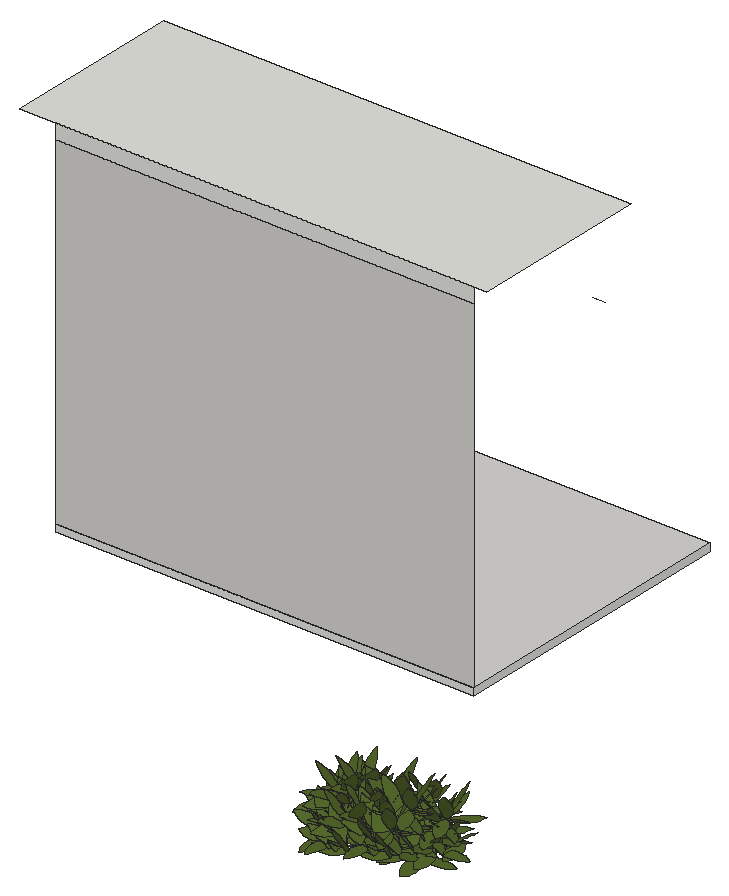
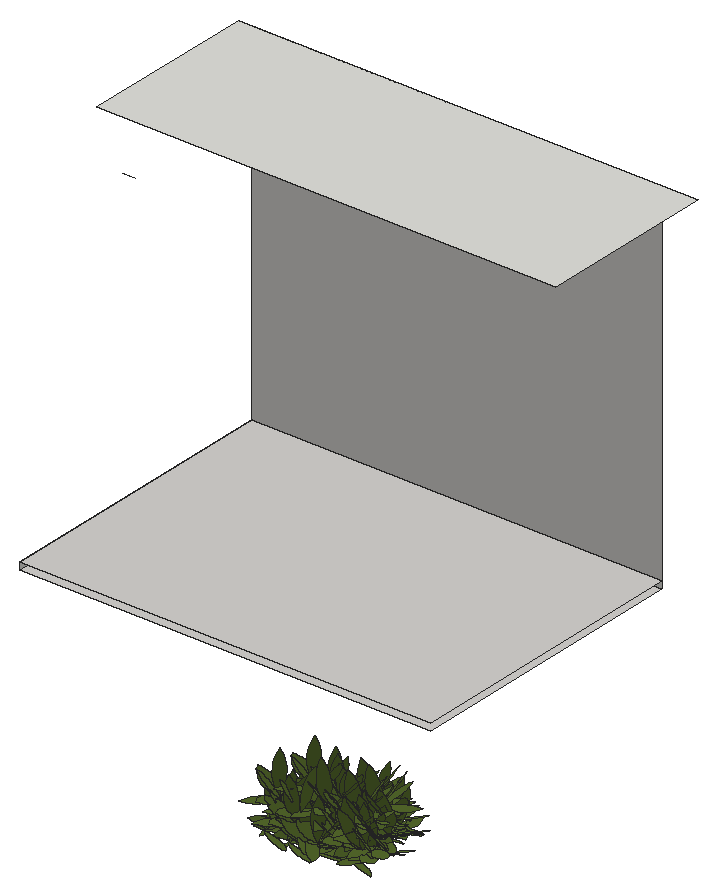
# SketchUp Ruby script. Lengths in inches.
U = 1.inch
M = Sketchup.active_model
def pt(a) = Geom::Point3d.new(a.map { |v| v * U })
def face(e, loops, mat)
  f = e.add_face(loops[0].map { |a| pt(a) })
  loops[1..].each { |l| e.add_face(l.map { |a| pt(a) }).erase! }
  f.material = f.back_material = mat if mat
  f
end
# faces: each face lists its corners as indices into pts; further lists are holes
def faces(e, pts, list, mat = nil) = list.each { |f| face(e, (f[0].is_a?(Array) ? f : [f]).map { |l| l.map { |i| pts[i] } }, mat) }
# xy, xz, yz: faces in a plane at the given z, y or x. An outline is a flat list of corners, or four numbers for a rectangle; further outlines are holes
def ring(l) = l.size == 4 ? [[l[0], l[1]], [l[2], l[1]], [l[2], l[3]], [l[0], l[3]]] : l.each_slice(2).to_a
def flat(e, list, mat, &to3) = list.each { |f| face(e, (f[0].is_a?(Array) ? f : [f]).map { |l| ring(l).map { |u, v| to3.(u, v) } }, mat) }
def xy(e, z, list, mat = nil) = flat(e, list, mat) { |x, y| [x, y, z] }
def xz(e, y, list, mat = nil) = flat(e, list, mat) { |x, z| [x, y, z] }
def yz(e, x, list, mat = nil) = flat(e, list, mat) { |y, z| [x, y, z] }
def lines(e, pts, list) = list.each { |a, b| e.add_line(pt(pts[a]), pt(pts[b])) }
# prism: a flat outline (further loops are holes) pulled along v
def prism(e, loops, v, mat = nil)
  f = face(e, loops, mat); d = Geom::Vector3d.new(v.map { |x| x * U })
  f.pushpull(f.normal.samedirection?(d) ? d.length : -d.length)
end
def box(e, o, s, mat = nil) = prism(e, [[o, [o[0] + s[0], o[1], o[2]], [o[0] + s[0], o[1] + s[1], o[2]], [o[0], o[1] + s[1], o[2]]]], [0, 0, s[2]], mat)
def at(x, y, z, deg = 0) = Geom::Transformation.translation(pt([x, y, z])) * Geom::Transformation.rotation(ORIGIN, Z_AXIS, deg.degrees)
def axes(o, x, y, z) = Geom::Transformation.new([*x, 0, *y, 0, *z, 0, *pt(o).to_a, 1])
def part(name) = M.definitions.add(name)
# library, detail: a bought-in or finely detailed component or shape, given as its bounding box
def library(name, o, s) = part(name).tap { |d| box(d.entities, o, s) }
def detail(e, o, s) = box(e.add_group.entities, o, s)
def put(e, d, t, mat = nil) = e.add_instance(d, t).tap { |i| i.material = mat if mat }
def group(e, t, mat = nil) = e.add_group.tap { |g| g.transformation = t; g.material = mat if mat }.entities
root = M.entities
M.materials.add("[0008_LavenderBlush]").color = [212, 210, 207]
M.materials.add("[Asphalt_New]").color = [85, 106, 44]
M.materials.add("white").color = [255, 255, 255]
c1 = part("Component\#59")
xy(c1.entities,0,[[5.79,0,4.75,0.06,3.73,0.22,2.73,0.5,1.77,0.88,0.86,1.37,0,1.95,0.83,2.59,1.74,3.13,2.7,3.56,3.7,3.87,4.74,4.05,5.79,4.12,6.84,4.05,7.87,3.87,8.88,3.56,9.84,3.13,10.74,2.59,11.57,1.95,10.72,1.37,9.8,0.88,8.84,0.5,7.84,0.22,6.82,0.06]],"[Asphalt_New]")
c2 = part("Leaf cluster")
put(c2.entities,c1,axes([10.37,9.23,1.73],[-0.67725,-0.67301,0.29729],[0.61625,-0.73963,-0.27052],[0.40195,0,0.91566]),"[Asphalt_New]")
put(c2.entities,c1,at(0,5.84,1.2),"[Asphalt_New]")
put(c2.entities,c1,axes([11.625,9.72,1.52],[-0.61694,-0.11161,0.77906],[-0.02647,-0.98639,-0.16227],[0.78657,-0.12073,0.60559]),"[Asphalt_New]")
put(c2.entities,c1,axes([13.35,8.05,1.98],[-0.1211,0.99122,-0.05316],[-0.90762,-0.13226,-0.39842],[-0.40195,0,0.91566]),"[Asphalt_New]")
c3 = part("Group141\#1")
p = [[0,0,0],[0,0,-2.45],[-0.68,0,-2.45],[4.45,-3.49,0],[-4.45,-3.49,0],[4.45,3.49,0],
  [4.45,0,0],[-4.45,3.49,0],[0.68,0,-2.45],[-4.45,0,0],[0,0,-3.97]]
lines(c3.entities,p,[[0,1],[1,2],[3,4],[5,6],[7,5],[1,8],[9,0],[0,6],[8,10],[4,9],[6,3],[2,10],
  [9,7]])
c4 = part("Rectangle Light")
put(c4.entities,c3,at(0,0,0))
xy(root,103.38,[[127.1875,9,148.875,24.3]],"[0008_LavenderBlush]")
xy(root,103.78,[[127.1875,9,148.875,24.3]],"[0008_LavenderBlush]")
xy(root,122.4375,[[125.3125,9,149.5625,18.35]])
xz(root,9,[[127.1875,103.38,148.875,103.78],[127.1875,121.625,148.875,122.4375]])
xz(root,9,[[127.1875,103.78,148.875,121.625]],"[0008_LavenderBlush]")
yz(root,148.875,[[9,103.38,24.3,103.78]])
p = [[148.875,16.67,118.57],[149.5625,16.67,118.57]]
lines(root,p,[[0,1]])
put(root,c1,axes([138.68,13.21,90.83],[0.01154,-0.09464,0.13861],[0.14952,-0.01265,-0.02887],[0.02521,0.11836,0.10775]),"[Asphalt_New]")
put(root,c1,axes([137.98,12,90.77],[0.00875,0.15182,0],[-0.15182,0.00875,0],[0,0,0.17792]),"[Asphalt_New]")
put(root,c1,axes([138.95,13.46,90.91],[-0.15155,-0.00971,-0.00946],[0.01213,-0.13895,-0.07089],[-0.00352,-0.06102,0.16292]),"[Asphalt_New]")
put(root,c1,axes([137.55,13.61,90.87],[0.09625,-0.10871,0.0529],[0.11768,0.08708,-0.04813],[0.00352,0.06102,0.16292]),"[Asphalt_New]")
put(root,c1,axes([137.45,12.3,90.56],[0.00875,0.15182,0],[-0.15182,0.00875,0],[0,0,0.17792]),"[Asphalt_New]")
put(root,c1,axes([137.49,13.8,90.83],[0.01154,-0.09464,0.13861],[0.14952,-0.01265,-0.02887],[0.02521,0.11836,0.10775]),"[Asphalt_New]")
put(root,c1,axes([139.68,12.39,90.99],[0.00875,0.15182,0],[-0.15182,0.00875,0],[0,0,0.17792]),"[Asphalt_New]")
put(root,c1,axes([140.28,13.99,90.83],[0.01154,-0.09464,0.13861],[0.14952,-0.01265,-0.02887],[0.02521,0.11836,0.10775]),"[Asphalt_New]")
put(root,c1,axes([137.02,13.91,90.65],[0.09625,-0.10871,0.0529],[0.11768,0.08708,-0.04813],[0.00352,0.06102,0.16292]),"[Asphalt_New]")
put(root,c1,axes([136.96,14.1,90.61],[0.01154,-0.09464,0.13861],[0.14952,-0.01265,-0.02887],[0.02521,0.11836,0.10775]),"[Asphalt_New]")
put(root,c2,axes([140.54,13.99,91.29],[-0.12016,0.09321,0],[-0.09321,-0.12016,0],[0,0,0.17792]),"white")
put(root,c1,axes([139.26,13.99,91.08],[0.09625,-0.10871,0.0529],[0.11768,0.08708,-0.04813],[0.00352,0.06102,0.16292]),"[Asphalt_New]")
put(root,c1,axes([139.19,14.19,91.04],[0.01154,-0.09464,0.13861],[0.14952,-0.01265,-0.02887],[0.02521,0.11836,0.10775]),"[Asphalt_New]")
put(root,c1,axes([139.41,12.8,90.77],[0.00875,0.15182,0],[-0.15182,0.00875,0],[0,0,0.17792]),"[Asphalt_New]")
put(root,c1,axes([137.76,14.05,90.91],[-0.15155,-0.00971,-0.00946],[0.01213,-0.13895,-0.07089],[-0.00352,-0.06102,0.16292]),"[Asphalt_New]")
put(root,c2,axes([137.56,12.1,91.42],[0.12994,0.079,0],[-0.079,0.12994,0],[0,0,0.17792]),"white")
put(root,c2,axes([141.87,13.48,91.41],[-0.06499,0.13748,0],[-0.13748,-0.06499,0],[0,0,0.17792]),"white")
put(root,c2,axes([136.61,13.25,90.73],[0.1271,-0.08349,0],[0.08349,0.1271,0],[0,0,0.17792]),"white")
put(root,c1,axes([139.68,14.6,91.41],[-0.12443,-0.07482,0.0529],[0.06418,-0.13158,-0.04813],[0.05936,-0.01458,0.16292]),"[Asphalt_New]")
put(root,c1,axes([140.55,14.24,90.91],[-0.15155,-0.00971,-0.00946],[0.01213,-0.13895,-0.07089],[-0.00352,-0.06102,0.16292]),"[Asphalt_New]")
put(root,c1,axes([138.98,14.4,90.87],[0.09625,-0.10871,0.0529],[0.11768,0.08708,-0.04813],[0.00352,0.06102,0.16292]),"[Asphalt_New]")
put(root,c1,axes([138.18,13.11,90.77],[0.00875,0.15182,0],[-0.15182,0.00875,0],[0,0,0.17792]),"[Asphalt_New]")
put(root,c1,axes([138.92,14.6,90.83],[0.01154,-0.09464,0.13861],[0.14952,-0.01265,-0.02887],[0.02521,0.11836,0.10775]),"[Asphalt_New]")
put(root,c1,axes([139.46,14.43,91.125],[-0.15155,-0.00971,-0.00946],[0.01213,-0.13895,-0.07089],[-0.00352,-0.06102,0.16292]),"[Asphalt_New]")
put(root,c1,axes([137.53,13.33,90.77],[0.00875,0.15182,0],[-0.15182,0.00875,0],[0,0,0.17792]),"[Asphalt_New]")
put(root,c1,axes([138.2,13.97,91.46],[0.15184,-0.00221,-0.00946],[-0.00119,0.13948,-0.07089],[0.0083,0.06056,0.16292]),"[Asphalt_New]")
put(root,c2,axes([141.41,13.92,91.41],[-0.06499,0.13748,0],[-0.13748,-0.06499,0],[0,0,0.17792]),"white")
put(root,c2,axes([138.25,15.96,90.87],[-0.12334,-0.08896,0],[0.08896,-0.12334,0],[0,0,0.17792]),"white")
put(root,c2,axes([140.5,14.72,90.51],[-0.12016,0.09321,0],[-0.09321,-0.12016,0],[0,0,0.17792]),"white")
put(root,c1,axes([137.76,14.71,90.87],[0.09625,-0.10871,0.0529],[0.11768,0.08708,-0.04813],[0.00352,0.06102,0.16292]),"[Asphalt_New]")
put(root,c1,axes([139.23,15.04,91.41],[-0.12443,-0.07482,0.0529],[0.06418,-0.13158,-0.04813],[0.05936,-0.01458,0.16292]),"[Asphalt_New]")
put(root,c1,axes([137.69,14.91,90.83],[0.01154,-0.09464,0.13861],[0.14952,-0.01265,-0.02887],[0.02521,0.11836,0.10775]),"[Asphalt_New]")
put(root,c1,axes([138.61,15.1875,91.18],[-0.09806,-0.10708,0.0529],[0.09891,-0.10794,-0.04813],[0.06106,0.00288,0.16292]),"[Asphalt_New]")
put(root,c1,axes([139.89,14.62,91.37],[-0.09516,0.0059,0.13861],[-0.03969,-0.14471,-0.02887],[0.11178,-0.04636,0.10775]),"[Asphalt_New]")
put(root,c2,axes([139.03,14.04,90.89],[-0.06499,0.13748,0],[-0.13748,-0.06499,0],[0,0,0.17792]),"white")
put(root,c2,axes([135.42,13.84,90.73],[0.1271,-0.08349,0],[0.08349,0.1271,0],[0,0,0.17792]),"white")
put(root,c2,axes([140.95,14.95,91.29],[-0.12303,0.08939,0],[-0.08939,-0.12303,0],[0,0,0.17792]),"white")
put(root,c2,axes([139.41,14.9,91.77],[-0.12016,0.09321,0],[-0.09321,-0.12016,0],[0,0,0.17792]),"white")
put(root,c1,axes([137.1,14.9375,90.87],[0.09625,-0.10871,0.0529],[0.11768,0.08708,-0.04813],[0.00352,0.06102,0.16292]),"[Asphalt_New]")
put(root,c1,axes([139.19,14.85,90.91],[-0.15155,-0.00971,-0.00946],[0.01213,-0.13895,-0.07089],[-0.00352,-0.06102,0.16292]),"[Asphalt_New]")
put(root,c2,axes([137.52,12.83,90.65],[0.12994,0.079,0],[-0.079,0.12994,0],[0,0,0.17792]),"white")
put(root,c2,axes([137.72,16.25,90.66],[-0.12334,-0.08896,0],[0.08896,-0.12334,0],[0,0,0.17792]),"white")
put(root,c1,axes([137.04,15.13,90.83],[0.01154,-0.09464,0.13861],[0.14952,-0.01265,-0.02887],[0.02521,0.11836,0.10775]),"[Asphalt_New]")
put(root,c1,axes([138.03,14.47,91.3125],[0.14768,-0.03627,0],[0.03627,0.14768,0],[0,0,0.17792]),"[Asphalt_New]")
put(root,c2,axes([141.01,14.73,91.18],[-0.10136,0.11337,0],[-0.11337,-0.10136,0],[0,0,0.17792]),"white")
put(root,c2,axes([138.21,14.03,90.73],[0.1271,-0.08349,0],[0.08349,0.1271,0],[0,0,0.17792]),"white")
put(root,c2,axes([142.32,14.29,92.12],[-0.06499,0.13748,0],[-0.13748,-0.06499,0],[0,0,0.17792]),"white")
put(root,c1,axes([138.04,15.48,91.18],[-0.09806,-0.10708,0.0529],[0.09891,-0.10794,-0.04813],[0.06106,0.00288,0.16292]),"[Asphalt_New]")
put(root,c2,axes([139.96,16.34,91.08],[-0.12334,-0.08896,0],[0.08896,-0.12334,0],[0,0,0.17792]),"white")
put(root,c2,axes([138.02,12.96,91.42],[0.12739,0.08305,0],[-0.08305,0.12739,0],[0,0,0.17792]),"white")
put(root,c2,axes([136.43,13.01,91.91],[0.12994,0.079,0],[-0.079,0.12994,0],[0,0,0.17792]),"white")
put(root,c1,axes([140.14,15.41,92.12],[-0.12443,-0.07482,0.0529],[0.06418,-0.13158,-0.04813],[0.05936,-0.01458,0.16292]),"[Asphalt_New]")
put(root,c1,axes([138.49,14.19,91.38],[-0.00408,0.09525,0.13861],[-0.14807,0.02435,-0.02887],[-0.03442,-0.11602,0.10775]),"[Asphalt_New]")
put(root,c1,axes([139.43,15.0625,91.37],[-0.09516,0.0059,0.13861],[-0.03969,-0.14471,-0.02887],[0.11178,-0.04636,0.10775]),"[Asphalt_New]")
put(root,c2,axes([137.13,14.22,90.95],[0.1271,-0.08349,0],[0.08349,0.1271,0],[0,0,0.17792]),"white")
put(root,c2,axes([138.56,15.26,91.0625],[-0.12016,0.09321,0],[-0.09321,-0.12016,0],[0,0,0.17792]),"white")
put(root,c1,axes([137.96,15.16,90.91],[-0.15155,-0.00971,-0.00946],[0.01213,-0.13895,-0.07089],[-0.00352,-0.06102,0.16292]),"[Asphalt_New]")
put(root,c1,axes([138.79,15.27,91.14],[-0.09292,-0.02137,0.13861],[0.00305,-0.15002,-0.02887],[0.12035,-0.0127,0.10775]),"[Asphalt_New]")
put(root,c1,axes([140.55,15.71,90.29],[0.01842,-0.15074,-0.00946],[0.13802,0.02011,-0.07089],[0.06112,0,0.16292]),"[Asphalt_New]")
put(root,c2,axes([140.45,15.03,91.18],[-0.10136,0.11337,0],[-0.11337,-0.10136,0],[0,0,0.17792]),"white")
put(root,c1,axes([139.51,15.73,90.5],[0.01842,-0.15074,-0.00946],[0.13802,0.02011,-0.07089],[0.06112,0,0.16292]),"[Asphalt_New]")
put(root,c1,axes([138.44,14.39,91.42],[-0.08742,0.11593,0.0529],[-0.12415,-0.07758,-0.04813],[-0.0083,-0.06056,0.16292]),"[Asphalt_New]")
put(root,c2,axes([140.89,13.39,90.11],[0.07604,0.1317,0],[-0.1317,0.07604,0],[0,0,0.17792]),"white")
put(root,c1,axes([137.05,14.6,91.08],[0.1519,0.00716,0],[-0.00716,0.1519,0],[0,0,0.17792]),"[Asphalt_New]")
put(root,c1,axes([138.16,14.6875,90.6875],[0.15184,-0.00221,-0.00946],[-0.00119,0.13948,-0.07089],[0.0083,0.06056,0.16292]),"[Asphalt_New]")
put(root,c2,axes([139.86,13.41,90.32],[0.07604,0.1317,0],[-0.1317,0.07604,0],[0,0,0.17792]),"white")
put(root,c2,axes([140.3,16.65,91.27],[-0.10525,-0.10976,0],[0.10976,-0.10525,0],[0,0,0.17792]),"white")
put(root,c1,axes([137.58,14.91,91.3125],[0.14768,-0.03627,0],[0.03627,0.14768,0],[0,0,0.17792]),"[Asphalt_New]")
put(root,c2,axes([139.6875,16.75,90.87],[-0.12334,-0.08896,0],[0.08896,-0.12334,0],[0,0,0.17792]),"white")
put(root,c1,axes([138.14,16.02,91.32],[-0.02064,-0.15066,0],[0.15066,-0.02064,0],[0,0,0.17792]),"[Asphalt_New]")
put(root,c1,axes([138.23,15.5625,91.14],[-0.09292,-0.02137,0.13861],[0.00305,-0.15002,-0.02887],[0.12035,-0.0127,0.10775]),"[Asphalt_New]")
put(root,c1,axes([138.61,14.85,91.46],[0.15183,0.00256,-0.00946],[-0.00557,0.13937,-0.07089],[0.00639,0.06079,0.16292]),"[Asphalt_New]")
put(root,c1,axes([137.07,14.875,91.95],[0.15184,-0.00221,-0.00946],[-0.00119,0.13948,-0.07089],[0.0083,0.06056,0.16292]),"[Asphalt_New]")
put(root,c2,axes([140.89,15.67,90.51],[-0.12303,0.08939,0],[-0.08939,-0.12303,0],[0,0,0.17792]),"white")
put(root,c1,axes([140.34,15.4375,92.08],[-0.09516,0.0059,0.13861],[-0.03969,-0.14471,-0.02887],[0.11178,-0.04636,0.10775]),"[Asphalt_New]")
put(root,c1,axes([140.08,14.3125,91.45],[0.01807,0.15078,-0.00946],[-0.13884,0.01339,-0.07089],[-0.05936,0.01458,0.16292]),"[Asphalt_New]")
put(root,c2,axes([136.85,14.64,90.73],[0.1271,-0.08349,0],[0.08349,0.1271,0],[0,0,0.17792]),"white")
put(root,c1,axes([136.49,14.89,91.08],[0.1519,0.00716,0],[-0.00716,0.1519,0],[0,0,0.17792]),"[Asphalt_New]")
put(root,c1,axes([138.81,16.09,91.89],[-0.09806,-0.10708,0.0529],[0.09891,-0.10794,-0.04813],[0.06106,0.00288,0.16292]),"[Asphalt_New]")
put(root,c2,axes([138.95,15.76,91.0625],[-0.12016,0.09321,0],[-0.09321,-0.12016,0],[0,0,0.17792]),"white")
put(root,c2,axes([139.79,15.82,91.77],[-0.12303,0.08939,0],[-0.08939,-0.12303,0],[0,0,0.17792]),"white")
put(root,c2,axes([138.46,17.0625,90.87],[-0.12334,-0.08896,0],[0.08896,-0.12334,0],[0,0,0.17792]),"white")
put(root,c1,axes([138.48,15.28,92.03],[0.14768,-0.03627,0],[0.03627,0.14768,0],[0,0,0.17792]),"[Asphalt_New]")
put(root,c2,axes([137.96,13.69,90.65],[0.12739,0.08305,0],[-0.08305,0.12739,0],[0,0,0.17792]),"white")
put(root,c2,axes([139.42,15.08,91.1],[-0.06499,0.13748,0],[-0.13748,-0.06499,0],[0,0,0.17792]),"white")
put(root,c2,axes([139.84,17.09,91.27],[-0.10525,-0.10976,0],[0.10976,-0.10525,0],[0,0,0.17792]),"white")
put(root,c1,axes([140.82,16.25,90.5],[0.01842,-0.15074,-0.00946],[0.13802,0.02011,-0.07089],[0.06112,0,0.16292]),"[Asphalt_New]")
put(root,c1,axes([140.45,14.56,91.3],[0.00875,0.15182,0],[-0.15182,0.00875,0],[0,0,0.17792]),"[Asphalt_New]")
put(root,c2,axes([141.22,15.64,91.89],[-0.10136,0.11337,0],[-0.11337,-0.10136,0],[0,0,0.17792]),"white")
put(root,c1,axes([137.24,16.19,91.1],[-0.12443,-0.07482,0.0529],[0.06418,-0.13158,-0.04813],[0.05936,-0.01458,0.16292]),"[Asphalt_New]")
put(root,c2,axes([141.16,13.93,90.32],[0.07604,0.1317,0],[-0.1317,0.07604,0],[0,0,0.17792]),"white")
put(root,c1,axes([136.21,15.24,91.24],[0.15184,-0.00221,-0.00946],[-0.00119,0.13948,-0.07089],[0.0083,0.06056,0.16292]),"[Asphalt_New]")
put(root,c1,axes([138.45,14.91,90.61],[-0.00408,0.09525,0.13861],[-0.14807,0.02435,-0.02887],[-0.03442,-0.11602,0.10775]),"[Asphalt_New]")
put(root,c2,axes([135.63,14.95,90.73],[0.1271,-0.08349,0],[0.08349,0.1271,0],[0,0,0.17792]),"white")
put(root,c2,axes([136.86,13.84,91.91],[0.12739,0.08305,0],[-0.08305,0.12739,0],[0,0,0.17792]),"white")
put(root,c2,axes([137.46,17.21,90.75],[-0.10525,-0.10976,0],[0.10976,-0.10525,0],[0,0,0.17792]),"white")
put(root,c1,axes([139.7,16.39,90.5],[0.01842,-0.15074,-0.00946],[0.13802,0.02011,-0.07089],[0.06112,0,0.16292]),"[Asphalt_New]")
put(root,c4,at(137.45,15.57,103.375,180))
put(root,c2,axes([137.81,17.29,90.87],[-0.12334,-0.08896,0],[0.08896,-0.12334,0],[0,0,0.17792]),"white")
put(root,c2,axes([139.875,15.27,90.89],[-0.06499,0.13748,0],[-0.13748,-0.06499,0],[0,0,0.17792]),"white")
put(root,c1,axes([138.4,15.11,90.64],[-0.08742,0.11593,0.0529],[-0.12415,-0.07758,-0.04813],[-0.0083,-0.06056,0.16292]),"[Asphalt_New]")
put(root,c2,axes([140.04,14.07,90.32],[0.07604,0.1317,0],[-0.1317,0.07604,0],[0,0,0.17792]),"white")
put(root,c2,axes([138.92,16.15,91.0625],[-0.12303,0.08939,0],[-0.08939,-0.12303,0],[0,0,0.17792]),"white")
put(root,c1,axes([139.625,14.76,91.45],[0.01807,0.15078,-0.00946],[-0.13884,0.01339,-0.07089],[-0.05936,0.01458,0.16292]),"[Asphalt_New]")
put(root,c2,axes([143.34,15.32,91.63],[-0.06499,0.13748,0],[-0.13748,-0.06499,0],[0,0,0.17792]),"white")
put(root,c1,axes([138.89,15.08,91.38],[-0.00707,0.09508,0.13861],[-0.14876,0.01968,-0.02887],[-0.03076,-0.11704,0.10775]),"[Asphalt_New]")
put(root,c1,axes([137.7,16.39,90.88],[-0.12443,-0.07482,0.0529],[0.06418,-0.13158,-0.04813],[0.05936,-0.01458,0.16292]),"[Asphalt_New]")
put(root,c2,axes([142.62,15.36,90.86],[-0.06499,0.13748,0],[-0.13748,-0.06499,0],[0,0,0.17792]),"white")
put(root,c1,axes([137.36,15.1,91.87],[-0.00408,0.09525,0.13861],[-0.14807,0.02435,-0.02887],[-0.03442,-0.11602,0.10775]),"[Asphalt_New]")
put(root,c1,axes([140.03,16.16,91.39],[0.09625,-0.10871,0.0529],[0.11768,0.08708,-0.04813],[0.00352,0.06102,0.16292]),"[Asphalt_New]")
put(root,c1,axes([142.58,16.04,90.15],[-0.15207,0,0],[0,-0.15207,0],[0,0,0.17792]),"[Asphalt_New]")
put(root,c2,axes([138.6,15.89,90.66],[-0.10136,0.11337,0],[-0.11337,-0.10136,0],[0,0,0.17792]),"white")
put(root,c1,axes([141.16,16.4375,91.63],[-0.12443,-0.07482,0.0529],[0.06418,-0.13158,-0.04813],[0.05936,-0.01458,0.16292]),"[Asphalt_New]")
put(root,c1,axes([138.99,16.18,91.85],[-0.09292,-0.02137,0.13861],[0.00305,-0.15002,-0.02887],[0.12035,-0.0127,0.10775]),"[Asphalt_New]")
put(root,c2,axes([134.98,15.17,90.73],[0.1271,-0.08349,0],[0.08349,0.1271,0],[0,0,0.17792]),"white")
put(root,c1,axes([141.54,16.07,90.36],[-0.15207,0,0],[0,-0.15207,0],[0,0,0.17792]),"[Asphalt_New]")
put(root,c1,axes([138.83,15.28,91.42],[-0.09102,0.11312,0.0529],[-0.12166,-0.08144,-0.04813],[-0.00639,-0.06079,0.16292]),"[Asphalt_New]")
put(root,c1,axes([140.43,16.48,90.86],[-0.12443,-0.07482,0.0529],[0.06418,-0.13158,-0.04813],[0.05936,-0.01458,0.16292]),"[Asphalt_New]")
put(root,c1,axes([137.25,14.88,90.93],[0.01807,0.15078,-0.00946],[-0.13884,0.01339,-0.07089],[-0.05936,0.01458,0.16292]),"[Asphalt_New]")
put(root,c1,axes([139.97,16.35,91.35],[0.01154,-0.09464,0.13861],[0.14952,-0.01265,-0.02887],[0.02521,0.11836,0.10775]),"[Asphalt_New]")
put(root,c2,axes([140.75,17.46,91.99],[-0.10525,-0.10976,0],[0.10976,-0.10525,0],[0,0,0.17792]),"white")
put(root,c2,axes([138.61,17.33,91.04],[-0.06975,-0.13513,0],[0.13513,-0.06975,0],[0,0,0.17792]),"white")
put(root,c1,axes([137.31,15.3,91.91],[-0.08742,0.11593,0.0529],[-0.12415,-0.07758,-0.04813],[-0.0083,-0.06056,0.16292]),"[Asphalt_New]")
put(root,c1,axes([138.1,16.75,90.55],[-0.02064,-0.15066,0],[0.15066,-0.02064,0],[0,0,0.17792]),"[Asphalt_New]")
put(root,c1,axes([139.07,15.03,91.22],[-0.0255,0.1497,-0.00946],[-0.13692,-0.02659,-0.07089],[-0.06106,-0.00288,0.16292]),"[Asphalt_New]")
put(root,c1,axes([137.26,15.5,91.79],[0.1519,0.00716,0],[-0.00716,0.1519,0],[0,0,0.17792]),"[Asphalt_New]")
put(root,c1,axes([140.8125,15.45,90.2],[0.09382,0.01697,0.13861],[0.00402,0.15,-0.02887],[-0.11961,0.01836,0.10775]),"[Asphalt_New]")
put(root,c1,axes([138.54,15.57,90.6875],[0.15183,0.00256,-0.00946],[-0.00557,0.13937,-0.07089],[0.00639,0.06079,0.16292]),"[Asphalt_New]")
put(root,c1,axes([139.78,15.48,90.42],[0.09382,0.01697,0.13861],[0.00402,0.15,-0.02887],[-0.11961,0.01836,0.10775]),"[Asphalt_New]")
put(root,c1,axes([136.59,16.76,91.25],[0.01842,-0.15074,-0.00946],[0.13802,0.02011,-0.07089],[0.06112,0,0.16292]),"[Asphalt_New]")
put(root,c1,axes([137.44,16.22,91.06],[-0.09516,0.0059,0.13861],[-0.03969,-0.14471,-0.02887],[0.11178,-0.04636,0.10775]),"[Asphalt_New]")
put(root,c1,axes([140.81,15.08,91.3],[0.00875,0.15182,0],[-0.15182,0.00875,0],[0,0,0.17792]),"[Asphalt_New]")
put(root,c1,axes([138.48,16.9,91.32],[-0.0159,-0.15124,0],[0.15124,-0.0159,0],[0,0,0.17792]),"[Asphalt_New]")
put(root,c1,axes([136.61,15.74,91.24],[0.15184,-0.00221,-0.00946],[-0.00119,0.13948,-0.07089],[0.0083,0.06056,0.16292]),"[Asphalt_New]")
put(root,c1,axes([137.01,16.93,91.8125],[-0.02064,-0.15066,0],[0.15066,-0.02064,0],[0,0,0.17792]),"[Asphalt_New]")
put(root,c1,axes([137.45,15.72,91.95],[0.15183,0.00256,-0.00946],[-0.00557,0.13937,-0.07089],[0.00639,0.06079,0.16292]),"[Asphalt_New]")
put(root,c1,axes([140.53,15.125,92.16],[0.01807,0.15078,-0.00946],[-0.13884,0.01339,-0.07089],[-0.05936,0.01458,0.16292]),"[Asphalt_New]")
put(root,c1,axes([137.3,16.9,90.47],[0.01842,-0.15074,-0.00946],[0.13802,0.02011,-0.07089],[0.06112,0,0.16292]),"[Asphalt_New]")
put(root,c2,axes([138.56,15.76,90.89],[-0.06499,0.13748,0],[-0.13748,-0.06499,0],[0,0,0.17792]),"white")
put(root,c2,axes([138.05,17.62,91.04],[-0.06975,-0.13513,0],[0.13513,-0.06975,0],[0,0,0.17792]),"white")
put(root,c1,axes([138.5,15.32,91.22],[-0.0255,0.1497,-0.00946],[-0.13692,-0.02659,-0.07089],[-0.06106,-0.00288,0.16292]),"[Asphalt_New]")
put(root,c2,axes([137.64,14.58,90.3],[0.07604,0.1317,0],[-0.1317,0.07604,0],[0,0,0.17792]),"white")
put(root,c1,axes([137.9,16.41,90.85],[-0.09516,0.0059,0.13861],[-0.03969,-0.14471,-0.02887],[0.11178,-0.04636,0.10775]),"[Asphalt_New]")
put(root,c2,axes([139.3,16.67,91.0625],[-0.12303,0.08939,0],[-0.08939,-0.12303,0],[0,0,0.17792]),"white")
put(root,c2,axes([138.62,16.09,90.24],[0.09591,-0.11801,0],[0.11801,0.09591,0],[0,0,0.17792]),"white")
put(root,c2,axes([137.58,16.11,90.46],[0.09591,-0.11801,0],[0.11801,0.09591,0],[0,0,0.17792]),"white")
put(root,c1,axes([141.36,16.46,91.59],[-0.09516,0.0059,0.13861],[-0.03969,-0.14471,-0.02887],[0.11178,-0.04636,0.10775]),"[Asphalt_New]")
put(root,c1,axes([140.64,16.5,90.82],[-0.09516,0.0059,0.13861],[-0.03969,-0.14471,-0.02887],[0.11178,-0.04636,0.10775]),"[Asphalt_New]")
put(root,c1,axes([140.38,16.6875,91.39],[0.09625,-0.10871,0.0529],[0.11768,0.08708,-0.04813],[0.00352,0.06102,0.16292]),"[Asphalt_New]")
put(root,c1,axes([140.24,16.6,91.44],[-0.15155,-0.00971,-0.00946],[0.01213,-0.13895,-0.07089],[-0.00352,-0.06102,0.16292]),"[Asphalt_New]")
put(root,c1,axes([139.93,15.38,92.01],[0.00875,0.15182,0],[-0.15182,0.00875,0],[0,0,0.17792]),"[Asphalt_New]")
put(root,c1,axes([142.84,16.59,90.36],[-0.15207,0,0],[0,-0.15207,0],[0,0,0.17792]),"[Asphalt_New]")
put(root,c2,axes([141.96,16.75,90.54],[-0.12016,0.09321,0],[-0.09321,-0.12016,0],[0,0,0.17792]),"white")
put(root,c1,axes([140.32,16.88,91.35],[0.01154,-0.09464,0.13861],[0.14952,-0.01265,-0.02887],[0.02521,0.11836,0.10775]),"[Asphalt_New]")
put(root,c1,axes([141,15.52,90.24],[0.10299,0.10235,0.0529],[-0.09371,0.11248,-0.04813],[-0.06112,0,0.16292]),"[Asphalt_New]")
put(root,c1,axes([136.04,16.26,90.79],[0.14768,-0.03627,0],[0.03627,0.14768,0],[0,0,0.17792]),"[Asphalt_New]")
put(root,c1,axes([136.58,16.05,91.24],[0.15183,0.00256,-0.00946],[-0.00557,0.13937,-0.07089],[0.00639,0.06079,0.16292]),"[Asphalt_New]")
put(root,c1,axes([138.79,17.2,90.625],[-0.09806,-0.10708,0.0529],[0.09891,-0.10794,-0.04813],[0.06106,0.00288,0.16292]),"[Asphalt_New]")
put(root,c1,axes([139.97,15.55,90.46],[0.10299,0.10235,0.0529],[-0.09371,0.11248,-0.04813],[-0.06112,0,0.16292]),"[Asphalt_New]")
put(root,c1,axes([138.82,15.48,90.75],[0.00875,0.15182,0],[-0.15182,0.00875,0],[0,0,0.17792]),"[Asphalt_New]")
put(root,c1,axes([138.82,15.8,90.61],[-0.00707,0.09508,0.13861],[-0.14876,0.01968,-0.02887],[-0.03076,-0.11704,0.10775]),"[Asphalt_New]")
put(root,c1,axes([141.08,16,90.42],[0.09382,0.01697,0.13861],[0.00402,0.15,-0.02887],[-0.11961,0.01836,0.10775]),"[Asphalt_New]")
put(root,c1,axes([139.5,16.3125,91.54],[0.14768,-0.03627,0],[0.03627,0.14768,0],[0,0,0.17792]),"[Asphalt_New]")
put(root,c1,axes([141.73,16.73,90.36],[-0.15207,0,0],[0,-0.15207,0],[0,0,0.17792]),"[Asphalt_New]")
put(root,c1,axes([138.78,16.35,90.76],[0.14768,-0.03627,0],[0.03627,0.14768,0],[0,0,0.17792]),"[Asphalt_New]")
put(root,c1,axes([138.77,16,90.64],[-0.09102,0.11312,0.0529],[-0.12166,-0.08144,-0.04813],[-0.00639,-0.06079,0.16292]),"[Asphalt_New]")
put(root,c1,axes([139.49,17.37,91.4],[-0.09806,-0.10708,0.0529],[0.09891,-0.10794,-0.04813],[0.06106,0.00288,0.16292]),"[Asphalt_New]")
put(root,c1,axes([139.5,16.98,92.1],[0.09625,-0.10871,0.0529],[0.11768,0.08708,-0.04813],[0.00352,0.06102,0.16292]),"[Asphalt_New]")
put(root,c1,axes([137.73,15.95,91.87],[-0.00707,0.09508,0.13861],[-0.14876,0.01968,-0.02887],[-0.03076,-0.11704,0.10775]),"[Asphalt_New]")
put(root,c1,axes([139.96,16.14,90.42],[0.09382,0.01697,0.13861],[0.00402,0.15,-0.02887],[-0.11961,0.01836,0.10775]),"[Asphalt_New]")
put(root,c2,axes([138.97,14.86,90.67],[0.12994,0.079,0],[-0.079,0.12994,0],[0,0,0.17792]),"white")
put(root,c1,axes([136.89,15.96,91.16],[-0.00408,0.09525,0.13861],[-0.14807,0.02435,-0.02887],[-0.03442,-0.11602,0.10775]),"[Asphalt_New]")
put(root,c2,axes([137.85,18.25,90.96],[-0.10525,-0.10976,0],[0.10976,-0.10525,0],[0,0,0.17792]),"white")
put(root,c2,axes([141.33,17.03,90.54],[-0.12016,0.09321,0],[-0.09321,-0.12016,0],[0,0,0.17792]),"white")
put(root,c2,axes([141.2,16.75,90.63],[-0.10136,0.11337,0],[-0.11337,-0.10136,0],[0,0,0.17792]),"white")
put(root,c1,axes([139.4375,17.18,92.06],[0.01154,-0.09464,0.13861],[0.14952,-0.01265,-0.02887],[0.02521,0.11836,0.10775]),"[Asphalt_New]")
put(root,c1,axes([138.4,17.08,90.84],[0.09625,-0.10871,0.0529],[0.11768,0.08708,-0.04813],[0.00352,0.06102,0.16292]),"[Asphalt_New]")
put(root,c1,axes([137.67,16.15,91.91],[-0.09102,0.11312,0.0529],[-0.12166,-0.08144,-0.04813],[-0.00639,-0.06079,0.16292]),"[Asphalt_New]")
put(root,c2,axes([135.8125,18.17,90.73],[-0.06975,-0.13513,0],[0.13513,-0.06975,0],[0,0,0.17792]),"white")
put(root,c1,axes([141.34,17.48,90.5],[0.01842,-0.15074,-0.00946],[0.13802,0.02011,-0.07089],[0.06112,0,0.16292]),"[Asphalt_New]")
put(root,c1,axes([138.34,17.28,90.8],[0.01154,-0.09464,0.13861],[0.14952,-0.01265,-0.02887],[0.02521,0.11836,0.10775]),"[Asphalt_New]")
put(root,c2,axes([138.8125,18.24,91.76],[-0.06975,-0.13513,0],[0.13513,-0.06975,0],[0,0,0.17792]),"white")
put(root,c2,axes([138.88,16.64,90.46],[0.09591,-0.11801,0],[0.11801,0.09591,0],[0,0,0.17792]),"white")
put(root,c1,axes([138.42,17.62,90.55],[-0.0159,-0.15124,0],[0.15124,-0.0159,0],[0,0,0.17792]),"[Asphalt_New]")
put(root,c2,axes([141.68,15.16,90.32],[0.07604,0.1317,0],[-0.1317,0.07604,0],[0,0,0.17792]),"white")
put(root,c1,axes([139.27,15.94,91.93],[-0.0255,0.1497,-0.00946],[-0.13692,-0.02659,-0.07089],[-0.06106,-0.00288,0.16292]),"[Asphalt_New]")
put(root,c2,axes([140.4,16.42,90.89],[-0.06499,0.13748,0],[-0.13748,-0.06499,0],[0,0,0.17792]),"white")
put(root,c2,axes([138.31,18.4375,90.75],[-0.10525,-0.10976,0],[0.10976,-0.10525,0],[0,0,0.17792]),"white")
put(root,c2,axes([141.9,16.92,91.4],[-0.10136,0.11337,0],[-0.11337,-0.10136,0],[0,0,0.17792]),"white")
put(root,c1,axes([138.62,17.1,91.11],[-0.15207,0,0],[0,-0.15207,0],[0,0,0.17792]),"[Asphalt_New]")
put(root,c1,axes([140.59,17.13,91.44],[-0.15155,-0.00971,-0.00946],[0.01213,-0.13895,-0.07089],[-0.00352,-0.06102,0.16292]),"[Asphalt_New]")
put(root,c1,axes([139.9375,17.64,90.5],[0.01842,-0.15074,-0.00946],[0.13802,0.02011,-0.07089],[0.06112,0,0.16292]),"[Asphalt_New]")
put(root,c2,axes([140.73,18.51,91.39],[-0.12334,-0.08896,0],[0.08896,-0.12334,0],[0,0,0.17792]),"white")
put(root,c1,axes([137.63,15.91,91.14],[0.01807,0.15078,-0.00946],[-0.13884,0.01339,-0.07089],[-0.05936,0.01458,0.16292]),"[Asphalt_New]")
put(root,c2,axes([141.77,18.49,91.5],[-0.10525,-0.10976,0],[0.10976,-0.10525,0],[0,0,0.17792]),"white")
put(root,c2,axes([138.34,15.14,90.67],[0.12994,0.079,0],[-0.079,0.12994,0],[0,0,0.17792]),"white")
put(root,c1,axes([138.22,17.54,90.88],[-0.12443,-0.07482,0.0529],[0.06418,-0.13158,-0.04813],[0.05936,-0.01458,0.16292]),"[Asphalt_New]")
put(root,c2,axes([137.77,16.78,90.46],[0.09591,-0.11801,0],[0.11801,0.09591,0],[0,0,0.17792]),"white")
put(root,c1,axes([138.98,17.28,90.59],[-0.09292,-0.02137,0.13861],[0.00305,-0.15002,-0.02887],[0.12035,-0.0127,0.10775]),"[Asphalt_New]")
put(root,c2,axes([141.05,18.53,90.72],[-0.10525,-0.10976,0],[0.10976,-0.10525,0],[0,0,0.17792]),"white")
put(root,c1,axes([137.33,17.77,91.8125],[-0.0159,-0.15124,0],[0.15124,-0.0159,0],[0,0,0.17792]),"[Asphalt_New]")
put(root,c1,axes([136.96,16.56,91.24],[0.15183,0.00256,-0.00946],[-0.00557,0.13937,-0.07089],[0.00639,0.06079,0.16292]),"[Asphalt_New]")
put(root,c2,axes([140.28,15.32,90.32],[0.07604,0.1317,0],[-0.1317,0.07604,0],[0,0,0.17792]),"white")
put(root,c1,axes([136.55,17.79,91.1],[-0.02064,-0.15066,0],[0.15066,-0.02064,0],[0,0,0.17792]),"[Asphalt_New]")
put(root,c1,axes([141.27,16.07,90.46],[0.10299,0.10235,0.0529],[-0.09371,0.11248,-0.04813],[-0.06112,0,0.16292]),"[Asphalt_New]")
put(root,c1,axes([136.85,16.51,91.17],[0.09382,0.01697,0.13861],[0.00402,0.15,-0.02887],[-0.11961,0.01836,0.10775]),"[Asphalt_New]")
put(root,c1,axes([139.33,17.23,90.34],[-0.15207,0,0],[0,-0.15207,0],[0,0,0.17792]),"[Asphalt_New]")
put(root,c2,axes([136.2,18.48,90.52],[-0.06975,-0.13513,0],[0.13513,-0.06975,0],[0,0,0.17792]),"white")
put(root,c1,axes([137.24,16.61,90.53],[0.1519,0.00716,0],[-0.00716,0.1519,0],[0,0,0.17792]),"[Asphalt_New]")
